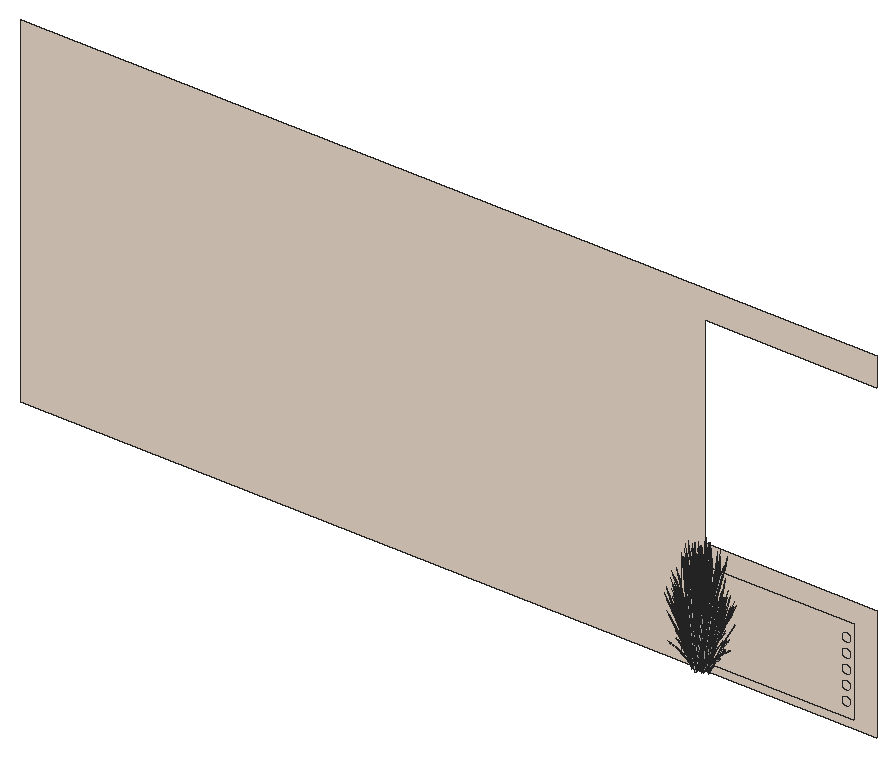
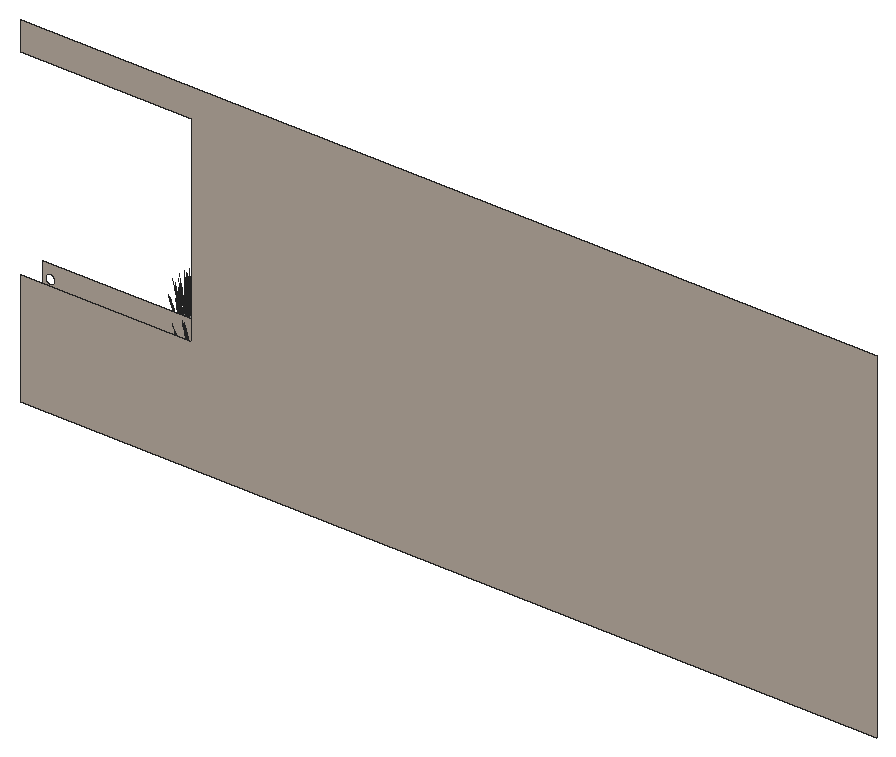
# SketchUp Ruby script. Lengths in inches.
U = 1.inch
M = Sketchup.active_model
def pt(a) = Geom::Point3d.new(a.map { |v| v * U })
def face(e, loops, mat)
  f = e.add_face(loops[0].map { |a| pt(a) })
  loops[1..].each { |l| e.add_face(l.map { |a| pt(a) }).erase! }
  f.material = f.back_material = mat if mat
  f
end
# faces: each face lists its corners as indices into pts; further lists are holes
def faces(e, pts, list, mat = nil) = list.each { |f| face(e, (f[0].is_a?(Array) ? f : [f]).map { |l| l.map { |i| pts[i] } }, mat) }
# xy, xz, yz: faces in a plane at the given z, y or x. An outline is a flat list of corners, or four numbers for a rectangle; further outlines are holes
def ring(l) = l.size == 4 ? [[l[0], l[1]], [l[2], l[1]], [l[2], l[3]], [l[0], l[3]]] : l.each_slice(2).to_a
def flat(e, list, mat, &to3) = list.each { |f| face(e, (f[0].is_a?(Array) ? f : [f]).map { |l| ring(l).map { |u, v| to3.(u, v) } }, mat) }
def xy(e, z, list, mat = nil) = flat(e, list, mat) { |x, y| [x, y, z] }
def xz(e, y, list, mat = nil) = flat(e, list, mat) { |x, z| [x, y, z] }
def yz(e, x, list, mat = nil) = flat(e, list, mat) { |y, z| [x, y, z] }
def lines(e, pts, list) = list.each { |a, b| e.add_line(pt(pts[a]), pt(pts[b])) }
# prism: a flat outline (further loops are holes) pulled along v
def prism(e, loops, v, mat = nil)
  f = face(e, loops, mat); d = Geom::Vector3d.new(v.map { |x| x * U })
  f.pushpull(f.normal.samedirection?(d) ? d.length : -d.length)
end
def box(e, o, s, mat = nil) = prism(e, [[o, [o[0] + s[0], o[1], o[2]], [o[0] + s[0], o[1] + s[1], o[2]], [o[0], o[1] + s[1], o[2]]]], [0, 0, s[2]], mat)
def at(x, y, z, deg = 0) = Geom::Transformation.translation(pt([x, y, z])) * Geom::Transformation.rotation(ORIGIN, Z_AXIS, deg.degrees)
def axes(o, x, y, z) = Geom::Transformation.new([*x, 0, *y, 0, *z, 0, *pt(o).to_a, 1])
def part(name) = M.definitions.add(name)
# library, detail: a bought-in or finely detailed component or shape, given as its bounding box
def library(name, o, s) = part(name).tap { |d| box(d.entities, o, s) }
def detail(e, o, s) = box(e.add_group.entities, o, s)
def put(e, d, t, mat = nil) = e.add_instance(d, t).tap { |i| i.material = mat if mat }
def group(e, t, mat = nil) = e.add_group.tap { |g| g.transformation = t; g.material = mat if mat }.entities
root = M.entities
M.materials.add("C01_Vanilla_Cream").color = [244, 228, 212]
M.materials.add("LightPink_Translucent").color = [144, 107, 117]
M.materials["LightPink_Translucent"].alpha = 0.75
c1 = part("blade")
p = [[2.15,0.21,22],[0,0.17,0],[0.09,0.45,0],[2.18,0.31,22],[2.29,0.31,22],[0.38,0.45,0],
  [2.48,0.24,33],[2.49,0.24,33],[2.48,0.22,33]]
faces(c1.entities,p,[[0,1,2,3],[4,5,2,3],[6,3,4,7],[8,0,3,6]])
c2 = part("seeds")
p = [[0.3,-0.1,1.38],[-0.01,-0.03,1.59],[-0.01,-0.03,0.03],[0.14,-0.07,-0.07],[0.29,-0.03,3],[0.15,0.01,3.11]]
faces(c2.entities,p,[[0,1,2,3],[1,0,4,5]],"LightPink_Translucent")
c3 = part("blade with seeds")
put(c3.entities,c1,at(0,0,0))
put(c3.entities,c2,axes([2.4,0.25,30.99],[1.5799,-0.05474,1.17369],[-0.12525,1.92788,0.29478],[-0.07173,-0.02425,1.56792]))
xz(root,468,[[[288,462,360,498],[357,490,356.48,490.07,356,490.27,355.59,490.59,355.27,491,355.07,491.48,355,492,355.07,492.52,355.27,493,355.59,493.41,356,493.73,356.48,493.93,357,494,357.52,493.93,358,493.73,358.41,493.41,358.73,493,358.93,492.52,359,492,358.93,491.48,358.73,491,358.41,490.59,358,490.27,357.52,490.07],[357,484,356.48,484.07,356,484.27,355.59,484.59,355.27,485,355.07,485.48,355,486,355.07,486.52,355.27,487,355.59,487.41,356,487.73,356.48,487.93,357,488,357.52,487.93,358,487.73,358.41,487.41,358.73,487,358.93,486.52,359,486,358.93,485.48,358.73,485,358.41,484.59,358,484.27,357.52,484.07],[357,478,356.48,478.07,356,478.27,355.59,478.59,355.27,479,355.07,479.48,355,480,355.07,480.52,355.27,481,355.59,481.41,356,481.73,356.48,481.93,357,482,357.52,481.93,358,481.73,358.41,481.41,358.73,481,358.93,480.52,359,480,358.93,479.48,358.73,479,358.41,478.59,358,478.27,357.52,478.07],[357,472,356.48,472.07,356,472.27,355.59,472.59,355.27,473,355.07,473.48,355,474,355.07,474.52,355.27,475,355.59,475.41,356,475.73,356.48,475.93,357,476,357.52,475.93,358,475.73,358.41,475.41,358.73,475,358.93,474.52,359,474,358.93,473.48,358.73,473,358.41,472.59,358,472.27,357.52,472.07],[357,466,356.48,466.07,356,466.27,355.59,466.59,355.27,467,355.07,467.48,355,468,355.07,468.52,355.27,469,355.59,469.41,356,469.73,356.48,469.93,357,470,357.52,469.93,358,469.73,358.41,469.41,358.73,469,358.93,468.52,359,468,358.93,467.48,358.73,467,358.41,466.59,358,466.27,357.52,466.07]]],"C01_Vanilla_Cream")
xz(root,480,[[0,450,0,594,360,594,360,582,288,582,288,498,360,498,360,450]],"C01_Vanilla_Cream")
put(root,c3,axes([303.38,460.31,465.51],[-0.14302,-0.44985,-0.38324],[0.54163,-0.07869,-0.29685],[0.15522,-0.12083,0.7333]))
put(root,c3,axes([301.01,458.76,463.6],[-0.38473,0.28263,-0.02919],[-0.35252,-0.30954,-0.13237],[-0.02482,-0.08771,0.43661]))
put(root,c3,axes([299.11,458.9,465.54],[-0.11979,-0.00348,1.31208],[-0.38137,0.34775,-0.2075],[-0.20349,-0.07106,0.10523]))
put(root,c3,axes([303.63,460.63,465.78],[-0.515,-0.27165,-0.0912],[0.2967,-0.3934,-0.50621],[0.1455,-0.13675,0.76918]))
put(root,c3,axes([301.51,462.11,464.49],[0.48111,0.19866,1.13446],[-0.47133,0.42798,0.44862],[-0.21112,-0.25366,0.95105]))
put(root,c3,axes([300.5,459.43,465.79],[0.08599,0.39682,0.2656],[-0.49155,0.10478,-0.3429],[-0.13203,-0.11372,0.65611]))
put(root,c3,axes([298.99,460.74,463.51],[0,-0.49266,-0.37238],[0.62289,0,0],[0,-0.11221,1.18128]))
put(root,c3,axes([300.72,459.28,463.51],[0.52105,-0.24633,-0.37238],[0.31144,0.44171,0],[0.11867,-0.0561,1.18128]))
put(root,c3,axes([303.8125,460.13,463.94],[-0.19889,-0.01459,1.07251],[-0.20376,-0.39145,-0.23066],[0.24434,-0.11074,0.45856]))
put(root,c3,axes([299.02,459.68,465.82],[0.45978,-0.36358,0.40322],[0.39653,0.38611,0.33247],[-0.21571,-0.06707,0.83437]))
put(root,c3,axes([304.9,460.51,465.53],[-0.07272,-0.00374,1.33037],[-0.30197,-0.40092,-0.12571],[0.12127,-0.13182,0.23543]))
put(root,c3,axes([301.34,460.29,463.54],[0.375,-0.3703,-0.46765],[0.46584,0.33578,-0.12274],[0.15027,-0.09237,1.03225]))
put(root,c3,axes([304.04,459.41,464.07],[-0.18544,0.25079,0.86145],[-0.15939,-0.33694,0.63294],[0.15316,-0.08443,0.18974]))
put(root,c3,axes([303.78,460.35,465.39],[0.48462,-0.07041,-0.2656],[0.12797,0.4025,0.3429],[0.13888,-0.10811,0.65611]))
put(root,c3,axes([299.23,459.68,465.55],[0.02803,-0.37463,0.04823],[0.42332,0.01027,0.37966],[-0.16216,-0.0392,0.57892]))
put(root,c3,axes([300.6875,460.9375,463.66],[0.27012,-0.44393,-0.33554],[0.56127,0.21365,0.16149],[0,-0.10233,1.07733]))
put(root,c3,axes([299.07,459.8,465.39],[-0.31678,-0.30846,-0.2656],[0.36171,-0.29199,0.3429],[-0.18378,-0.04443,0.65611]))
put(root,c3,axes([300.93,460.72,464],[-0.06488,-0.56215,-0.21822],[0.6757,-0.03399,-0.37502],[0.11898,-0.07488,1.19781]))
put(root,c3,axes([299.26,460.75,463.52],[0.38863,-0.30738,-0.23233],[0.38863,0.30738,0.23233],[0,-0.09901,1.0423]))
put(root,c3,axes([299.1,459.27,463.6],[-0.1606,0.40228,-0.02919],[-0.4943,-0.12375,-0.13237],[-0.07505,-0.0658,0.43661]))
put(root,c3,axes([303.38,460.59,465.79],[-0.48462,0.07041,0.2656],[-0.12797,-0.4025,-0.3429],[0.13888,-0.10811,0.65611]))
put(root,c3,axes([300.62,461.31,464],[-0.62699,-0.23507,-0.21822],[0.3019,-0.49615,-0.37502],[-0.0197,-0.12182,1.19781]))
put(root,c3,axes([298.83,461.11,463.78],[-0.69617,0,0],[0,-0.55062,-0.38706],[0,-0.12541,1.22783]))
put(root,c3,axes([298.95,460.13,463.94],[0.1087,0.13716,1.07251],[-0.25048,0.37284,-0.23066],[-0.25719,-0.08912,0.45856]))
put(root,c3,axes([300.84,459.47,463.52],[0.51941,0.1219,-0.23233],[-0.13078,0.42928,0.23233],[0.10471,-0.0495,1.0423]))
put(root,c3,axes([299.4,460.01,465.74],[-0.55654,-0.01186,-0.53284],[0.03738,-0.49951,0.0643],[-0.23578,-0.05271,0.75375]))
put(root,c3,axes([303.82,460.53,465.55],[0.3822,0.20719,0.04823],[-0.22252,0.29505,0.37966],[0.12254,-0.09539,0.57892]))
put(root,c3,axes([303.71,460.44,465.55],[0.13808,0.45342,0.36002],[-0.54163,0.07869,0.29685],[0.15963,-0.10664,0.74497]))
put(root,c3,axes([305.18,460.99,465.54],[0.07726,-0.07504,1.31208],[-0.09888,-0.46032,-0.2075],[0.19384,-0.08728,0.10523]))
put(root,c3,axes([299.375,460.97,463.75],[-0.51786,0.4142,0.23067],[-0.51817,-0.40984,-0.27369],[-0.01808,-0.11762,1.23664]))
put(root,c3,axes([298.65,459.19,465.53],[0.04127,0.04917,1.33037],[-0.19898,0.44196,-0.12571],[-0.20151,0.0032,0.23543]))
put(root,c3,axes([301.02,461.16,463.82],[0.6273,0.23878,0.18048],[-0.3019,0.49615,0.37502],[0,-0.11437,1.20407]))
put(root,c3,axes([300.78,461.83,463.83],[0.14756,-0.58378,-0.17572],[0.69966,0.10176,0.38453],[-0.12225,-0.08062,1.1733]))
put(root,c3,axes([299.22,460.11,465.51],[-0.40426,0.32635,-0.38324],[-0.35404,-0.34474,-0.29685],[-0.2054,-0.04965,0.7333]))
put(root,c3,axes([299.52,459.96,465.79],[0.31678,0.30846,0.2656],[-0.36171,0.29199,-0.3429],[-0.18378,-0.04443,0.65611]))
put(root,c3,axes([298.31,460.54,464.07],[0.35544,-0.03525,0.86145],[-0.22547,0.31061,0.63294],[-0.17565,-0.04659,0.18974]))
put(root,c3,axes([300.82,460.83,464.04],[-0.60457,0.03041,0.33554],[-0.05467,-0.50484,-0.16149],[0.10823,-0.05117,1.07733]))
put(root,c3,axes([299.43,459.76,465.78],[-0.02981,0.50103,-0.0912],[-0.56442,-0.01369,-0.50621],[-0.21738,-0.0348,0.76918]))
put(root,c3,axes([299.26,461.19,463.86],[0,0.49266,0.37238],[-0.62289,0,0],[0,-0.11221,1.18128]))
put(root,c3,axes([303.65,461.6875,465.78],[-0.28012,-0.44611,-0.0912],[0.49717,-0.21923,-0.50621],[0.20951,-0.05886,0.76918]))
put(root,c3,axes([303.63,461.3,465.51],[0.15083,-0.44814,-0.38324],[0.51712,0.15361,-0.29685],[0.2082,-0.04109,0.7333]))
put(root,c3,axes([302.8125,459.48,463.78],[0.34808,-0.49367,0],[0.58235,0.27531,-0.38706],[0.13264,0.0627,1.22783]))
put(root,c3,axes([298.71,460.45,464.91],[0.23093,-0.01116,1.28532],[-0.15319,0.4836,0.10393],[-0.32909,-0.02991,0.54946]))
put(root,c3,axes([300.73,461.59,463.66],[-0.33445,-0.41351,-0.33554],[0.50659,-0.29119,0.16149],[-0.10823,-0.05117,1.07733]))
put(root,c3,axes([300.8,461.01,463.77],[0.24206,0.5509,0.34316],[-0.69162,0.19157,0.13466],[0.00845,-0.10123,1.19142]))
put(root,c3,axes([304.18,461.43,463.49],[-0.35858,0.05912,1.06187],[-0.05708,-0.47061,0.06078],[0.25115,-0.07123,0.60425]))
put(root,c3,axes([304.83,461.01,463.7],[-0.34516,-0.31503,-0.04866],[0.37803,-0.28865,-0.22062],[0.10711,-0.02032,0.72768]))
put(root,c3,axes([300.68,461.44,464.04],[-0.27012,0.44393,0.33554],[-0.56127,-0.21365,-0.16149],[0,-0.10233,1.07733]))
put(root,c3,axes([301.67,461.05,463.65],[0,-0.57005,0],[0.69617,0,0],[0,0,1.34592]))
put(root,c3,axes([302.51,459.74,463.86],[-0.52105,-0.24633,0.37238],[0.31144,-0.44171,0],[0.11867,0.0561,1.18128]))
put(root,c3,axes([303.53,461.47,465.74],[0.48922,-0.21758,-0.53284],[0.27264,0.44789,0.0643],[0.23638,-0.05088,0.75375]))
put(root,c3,axes([300.43,461.75,463.54],[-0.57914,-0.08077,-0.46765],[0.12221,-0.49823,-0.12274],[-0.17283,-0.06037,1.03225]))
put(root,c3,axes([301.34,460.7,463.77],[-0.46162,0.4471,0.34316],[-0.54842,-0.39467,0.13466],[0.11129,-0.04462,1.19142]))
put(root,c3,axes([301.84,461.5,463.72],[-0.51786,-0.42404,-0.04598],[0.51817,-0.4243,0],[-0.01808,-0.01481,1.31678]))
put(root,c3,axes([300.54,459.96,463.86],[-0.16083,0.48962,0.13232],[-0.58854,-0.13856,0.26315],[0.10167,-0.00238,1.20305]))
put(root,c3,axes([303.46,461.55,465.79],[-0.46269,-0.13744,0.2656],[0.13495,-0.40096,-0.3429],[0.18628,-0.03677,0.65611]))
put(root,c3,axes([298.62,460.82,465.55],[0.15729,-0.44921,0.36002],[0.51712,0.15361,0.29685],[-0.20336,0.027,0.74497]))
put(root,c3,axes([300.29,460.35,463.2],[-0.548,0.19724,0.96696],[-0.17442,-0.56594,0.37572],[0.3365,0.00941,1.09981]))
put(root,c3,axes([301.77,460.5,463.96],[0.1074,-0.43968,0.1086],[0.52474,0.07632,-0.3101],[0.0955,0.04515,0.95058]))
put(root,c3,axes([298.58,460.7,465.55],[-0.20448,-0.33592,0.04823],[0.37288,-0.16442,0.37966],[-0.16437,0.03244,0.57892]))
put(root,c3,axes([300.86,461.55,463.77],[0.70367,0.1038,0.34316],[-0.1432,0.58624,0.13466],[-0.10283,-0.05661,1.19142]))
put(root,c3,axes([304.57,461.125,463.12],[-0.0291,-0.0748,1.32257],[0.20181,-0.43752,-0.20205],[0.20357,-0.00629,0.22528]))
put(root,c3,axes([298.57,461.05,463.12],[0.01412,0.07764,1.32257],[-0.28464,0.40547,-0.20205],[-0.20218,-0.02044,0.22528]))
put(root,c3,axes([301.54,460.62,464.04],[-0.33445,-0.41351,0.33554],[0.50659,-0.29119,-0.16149],[0.10823,0.05117,1.07733]))
put(root,c3,axes([299.8125,462.51,463.52],[-0.13078,-0.42928,-0.23233],[0.51941,-0.1219,0.23233],[-0.10471,-0.0495,1.0423]))
put(root,c3,axes([300.48,462.48,463.86],[0.59825,-0.13076,0.13232],[0.14773,0.48663,0.26315],[-0.05336,-0.0709,1.20305]))
put(root,c3,axes([301.71,460.65,464],[0.56211,-0.32708,-0.21822],[0.3738,0.46216,-0.37502],[0.13869,0.04694,1.19781]))
put(root,c3,axes([303.95,461.51,465.39],[0.46269,0.13744,-0.2656],[-0.13495,0.40096,0.3429],[0.18628,-0.03677,0.65611]))
put(root,c3,axes([299.67,462.69,463.51],[-0.52105,-0.24633,-0.37238],[0.31144,-0.44171,0],[-0.11867,-0.0561,1.18128]))
put(root,c3,axes([303.13,459.78,463.51],[0.52105,0.24633,-0.37238],[-0.31144,0.44171,0],[0.11867,0.0561,1.18128]))
put(root,c3,axes([298.51,460.87,465.39],[-0.46269,-0.13744,-0.2656],[0.13495,-0.40096,0.3429],[-0.18628,0.03677,0.65611]))
put(root,c3,axes([302.14,461.18,463.65],[0.62289,0,0],[0,0.51004,0],[0,0,1.33805]))
put(root,c3,axes([301.08,461.82,464],[-0.56211,0.32708,-0.21822],[-0.3738,-0.46216,-0.37502],[-0.13869,-0.04694,1.19781]))
put(root,c3,axes([302.32,459.99,463.86],[-0.59825,0.13076,0.13232],[-0.14773,-0.48663,0.26315],[0.05336,0.0709,1.20305]))
put(root,c3,axes([302.6875,461.01,464.91],[-0.23093,0.01116,1.28532],[0.15319,-0.4836,0.10393],[0.32909,0.02991,0.54946]))
put(root,c3,axes([302.98,459.96,463.52],[0.13078,0.42928,-0.23233],[-0.51941,0.1219,0.23233],[0.10471,0.0495,1.0423]))
put(root,c3,axes([303.88,461.68,465.55],[0.20448,0.33592,0.04823],[-0.37288,0.16442,0.37966],[0.16437,-0.03244,0.57892]))
put(root,c3,axes([301.9375,460.92,463.79],[-0.70367,-0.1038,0.36899],[0.1432,-0.58624,0.1448],[0.10283,0.05661,1.2811]))
put(root,c3,axes([303.84,461.56,465.55],[-0.15729,0.44921,0.36002],[-0.51712,-0.15361,0.29685],[0.20336,-0.027,0.74497]))
put(root,c3,axes([301.38,462.37,463.65],[-0.18165,-0.42474,0],[0.51872,-0.14874,0],[0,0,1.15778]))
put(root,c3,axes([301.03,461.97,463.96],[-0.1074,0.43968,0.1086],[-0.52474,-0.07632,-0.3101],[-0.0955,-0.04515,0.95058]))
put(root,c3,axes([299,460.83,465.79],[0.46269,0.13744,0.2656],[-0.13495,0.40096,-0.3429],[-0.18628,0.03677,0.65611]))
put(root,c3,axes([302.06,462.31,463.64],[0.5845,-0.16716,-0.14398],[0.20539,0.48152,0.00006],[0.06452,-0.01848,1.30423]))
put(root,c3,axes([302.26,462.51,463.86],[0.16083,-0.48962,0.13232],[0.58854,0.13856,0.26315],[-0.10167,0.00238,1.20305]))
put(root,c3,axes([302.125,461.4,463.66],[0.38863,0.31822,0],[-0.38863,0.31822,0],[0,0,1.2695]))
put(root,c3,axes([299.92,460.8,464.51],[0.15825,-0.07127,1.32798],[0.05457,0.4976,0.10393],[-0.34278,0.06603,0.47463]))
put(root,c3,axes([303.18,461.26,463.86],[-0.43742,-0.35886,0.13232],[0.44081,-0.34807,0.26315],[-0.04831,0.07329,1.20305]))
put(root,c3,axes([302.37,460.72,463.54],[0.57914,0.08077,-0.46765],[-0.12221,0.49823,-0.12274],[0.17283,0.06037,1.03225]))
put(root,c3,axes([304.93,461.59,464.07],[-0.34399,0.08133,0.86145],[0.16192,-0.33614,0.63294],[0.18249,0.023,0.18974]))
put(root,c3,axes([301.25,462.5625,463.65],[-0.56127,-0.22118,0],[0.27012,-0.45959,0],[0,0,1.2203]))
put(root,c3,axes([301.72,461.97,463.85],[-0.54364,-0.39653,-0.18894],[0.45745,-0.44527,0.41347],[-0.14639,0.04639,1.26162]))
put(root,c3,axes([300.28,462.73,463.86],[0.52105,0.24633,0.37238],[-0.31144,0.44171,0],[-0.11867,-0.0561,1.18128]))
put(root,c3,axes([302.12,461.03,464.04],[0.27012,-0.44393,0.33554],[0.56127,0.21365,-0.16149],[0,0.10233,1.07733]))
put(root,c3,axes([304.77,463.01,465.53],[-0.05034,-0.04313,1.33037],[0.11012,-0.46232,-0.12571],[0.1983,-0.02954,0.23543]))
put(root,c3,axes([298.22,461.14,465.54],[-0.09091,0.06396,1.31208],[0.00773,0.46734,-0.2075],[-0.20839,0.06078,0.10523]))
put(root,c3,axes([302.02,461.28,463.72],[0,0.56976,-0.04228],[-0.69617,0,0],[0,0.01791,1.34526]))
put(root,c3,axes([298.83,461.07,465.51],[-0.15083,0.44814,-0.38324],[-0.51712,-0.15361,-0.29685],[-0.2082,0.04109,0.7333]))
put(root,c3,axes([298.8,460.69,465.78],[0.28012,0.44611,-0.0912],[-0.49717,0.21923,-0.50621],[-0.20951,0.05886,0.76918]))
put(root,c3,axes([302.07,460.88,463.66],[0.33445,0.41351,-0.33554],[-0.50659,0.29119,0.16149],[0.10823,0.05117,1.07733]))
put(root,c3,axes([304.33,462.625,464.95],[-0.10656,-0.41414,-0.02619],[0.50364,-0.09521,-0.11874],[0.10517,0.02626,0.39164]))
put(root,c3,axes([299.98,462.99,463.78],[-0.34808,0.49367,0],[-0.58235,-0.27531,-0.38706],[-0.13264,-0.0627,1.22783]))
put(root,c3,axes([303.02,462.61,465.78],[0.02981,-0.50103,-0.0912],[0.56442,0.01369,-0.50621],[0.21738,0.0348,0.76918]))
put(root,c3,axes([303.54,461.28,463.86],[0,-0.49266,0.37238],[0.62289,0,0],[0,0.11221,1.18128]))
put(root,c3,axes([301.98,461.64,464.04],[0.60457,-0.03041,0.33554],[0.05467,0.50484,-0.16149],[-0.10823,0.05117,1.07733]))
put(root,c3,axes([302.36,461.13,463.96],[0.51872,-0.14368,0.1086],[0.18165,0.41027,-0.3101],[0,0.09029,0.95058]))
put(root,c3,axes([302.9375,462.42,465.79],[-0.31678,-0.30846,0.2656],[0.36171,-0.29199,-0.3429],[0.18378,0.04443,0.65611]))
put(root,c3,axes([301.44,461.89,463.66],[-0.60457,0.03041,-0.33554],[-0.05467,-0.50484,0.16149],[-0.10823,0.05117,1.07733]))
put(root,c3,axes([304.28,462.13,463.94],[-0.13408,-0.12117,1.07251],[0.17446,-0.40083,-0.23066],[0.27128,0.0543,0.45856]))
put(root,c3,axes([301.89,462.57,463.65],[0.56127,0.22118,0],[-0.27012,0.45959,0],[0,0,1.31215]))
put(root,c3,axes([303.52,462.3125,465.54],[0.11943,-0.00833,1.31208],[0.32759,-0.38275,-0.2075],[0.21244,0.05052,0.10523]))
put(root,c3,axes([302.11,463.06,463.64],[-0.34375,-0.4954,-0.03857],[0.58235,-0.27531,0.38706],[-0.1435,0.04717,1.22723]))
put(root,c3,axes([301.99,461.86,463.96],[0.41131,0.296,0.1086],[-0.34309,0.33395,-0.3101],[-0.0955,0.04515,0.95058]))
put(root,c3,axes([298.74,461.9375,465.55],[-0.13808,-0.45342,0.36002],[0.54163,-0.07869,0.29685],[-0.15963,0.10664,0.74497]))
put(root,c3,axes([298.63,461.85,465.55],[-0.3822,-0.20719,0.04823],[0.22252,-0.29505,0.37966],[-0.12254,0.09539,0.57892]))
put(root,c3,axes([298.81,461.31,464.91],[0.19317,-0.10421,1.28532],[0.16263,0.48153,0.10393],[-0.30326,0.10883,0.54946]))
put(root,c3,axes([303.05,462.375,465.74],[0.55654,0.01186,-0.53284],[-0.03738,0.49951,0.0643],[0.23578,0.05271,0.75375]))
put(root,c3,axes([302.43,462.77,463.86],[0.52105,-0.24633,0.37238],[0.31144,0.44171,0],[-0.11867,0.0561,1.18128]))
put(root,c3,axes([301.68,462.38,463.72],[0.24206,0.56598,-0.04509],[-0.69162,0.19832,0],[0.00845,0.01976,1.2913]))
put(root,c3,axes([301.95,463,463.52],[-0.51941,-0.1219,-0.23233],[0.13078,-0.42928,0.23233],[-0.10471,0.0495,1.0423]))
put(root,c3,axes([298.21,462.125,463.94],[0.19348,0.04044,1.07251],[0.1247,0.41309,-0.23066],[-0.26282,0.07733,0.45856]))
put(root,c3,axes([299.07,461.79,465.79],[0.48462,-0.07041,0.2656],[0.12797,0.4025,-0.3429],[-0.13888,0.10811,0.65611]))
put(root,c3,axes([303.96,461.36,463.78],[0.69617,0,0],[0,0.55062,-0.38706],[0,0.12541,1.22783]))
put(root,c3,axes([297.21,461.61,465.53],[0.07105,0.01321,1.33037],[0.2198,0.43529,-0.12571],[-0.14545,0.11425,0.23543]))
put(root,c3,axes([303.68,461.64,463.65],[-0.69582,-0.00394,-0.03732],[0,-0.55062,0.37457],[-0.02187,0.12535,1.18764]))
put(root,c3,axes([302.18,461.16,464],[0.62699,0.23507,-0.21822],[-0.3019,0.49615,-0.37502],[0.0197,0.12182,1.19781]))
put(root,c3,axes([297.8,462.99,464.07],[0.23202,-0.22328,0.86145],[0.09155,0.35348,0.63294],[-0.16768,0.06329,0.18974]))
put(root,c3,axes([303.39,462.58,465.39],[0.31678,0.30846,-0.2656],[-0.36171,0.29199,0.3429],[0.18378,0.04443,0.65611]))
put(root,c3,axes([303.54,461.72,463.52],[-0.38863,0.30738,-0.23233],[-0.38863,-0.30738,0.23233],[0,0.09901,1.0423]))
put(root,c3,axes([301.86,461.75,464],[0.06488,0.56215,-0.21822],[-0.6757,0.03399,-0.37502],[-0.11898,0.07488,1.19781]))
put(root,c3,axes([303.23,462.7,465.55],[-0.02803,0.37463,0.04823],[-0.42332,-0.01027,0.37966],[0.16216,0.0392,0.57892]))
put(root,c3,axes([302.11,461.53,463.66],[-0.27012,0.44393,-0.33554],[-0.56127,-0.21365,0.16149],[0,0.10233,1.07733]))
put(root,c3,axes([298.68,462.03,465.39],[-0.48462,0.07041,-0.2656],[-0.12797,-0.4025,0.3429],[-0.13888,0.10811,0.65611]))
put(root,c3,axes([303.26,462.58,465.55],[-0.41051,0.32462,0.36002],[-0.35404,-0.34474,0.29685],[0.1926,0.05988,0.74497]))
put(root,c3,axes([297.97,462.93,466.23],[0.49129,0.13151,-0.04866],[-0.15113,0.40475,-0.22062],[-0.08035,0.06145,0.72768]))
put(root,c3,axes([301.46,462.18,463.54],[-0.375,0.3703,-0.46765],[-0.46584,-0.33578,-0.12274],[-0.15027,0.09237,1.03225]))
put(root,c3,axes([301.96,462.95,465.79],[-0.08599,-0.39682,0.2656],[0.49155,-0.10478,-0.3429],[0.13203,0.11372,0.65611]))
put(root,c3,axes([302.125,462.81,463.75],[0.697,0.16013,0.23067],[-0.17437,0.57237,-0.27369],[-0.11536,0.07164,1.23664]))
put(root,c3,axes([302.08,463.19,463.51],[-0.52105,0.24633,-0.37238],[-0.31144,-0.44171,0],[-0.11867,0.0561,1.18128]))
put(root,c3,axes([303.81,461.73,463.51],[0,0.49266,-0.37238],[-0.62289,0,0],[0,0.11221,1.18128]))
put(root,c3,axes([302.25,461.79,464.91],[-0.2068,-0.08488,1.28532],[0.42797,-0.35609,0.10393],[0.26673,0.16064,0.54946]))
put(root,c3,axes([302.29,460.67,465.36],[-0.48108,-0.25598,1.03712],[0.50798,-0.39855,0.44749],[0.15521,0.24018,1.00248]))
put(root,c3,axes([298.82,461.75,465.78],[0.515,0.27165,-0.0912],[-0.2967,0.3934,-0.50621],[-0.1455,0.13675,0.76918]))
put(root,c3,axes([303.02,462.76,464.07],[-0.31347,-0.14166,0.86145],[0.40476,-0.14393,0.63294],[0.10917,0.12192,0.18974]))
put(root,c3,axes([301.91,463.16,465.78],[0.33176,-0.4217,-0.0912],[0.48044,0.24295,-0.50621],[0.16701,0.11914,0.76918]))
put(root,c3,axes([299.51,461.63,464.91],[0.13906,-0.15138,1.28532],[0.35111,0.40859,0.10393],[-0.24082,0.18608,0.54946]))
put(root,c3,axes([299.08,462.07,465.51],[0.14302,0.44985,-0.38324],[-0.54163,0.07869,-0.29685],[-0.15522,0.12083,0.7333]))
put(root,c3,axes([299.73,462.59,465.79],[0.3767,-0.25939,0.2656],[0.3566,0.29618,-0.3429],[-0.05426,0.15048,0.65611]))
put(root,c3,axes([302.55,463.12,463.78],[0.34808,0.49367,0],[-0.58235,0.27531,-0.38706],[-0.13264,0.0627,1.22783]))
put(root,c3,axes([301.48,463.51,465.53],[0.00165,-0.05965,1.33037],[0.47711,-0.26315,-0.12571],[0.16572,0.09393,0.23543]))
put(root,c3,axes([303.1,463.28,463.12],[0.04056,-0.07113,1.32257],[0.51066,-0.20948,-0.20205],[0.15482,0.10842,0.22528]))
put(root,c3,axes([302.25,461.16,464.13],[-0.01521,-0.46386,1.05954],[0.68831,0.12024,0.44862],[-0.1628,0.25382,1.00012]))
put(root,c3,axes([302.43,461.67,463.57],[0.20414,0.45107,-0.51909],[-0.58805,0.16245,-0.13624],[0.02256,0.15274,1.1458]))
put(root,c3,axes([299.39,462.83,465.55],[-0.45752,-0.02296,0.04823],[0.01254,-0.34663,0.37966],[-0.04787,0.13278,0.57892]))
put(root,c3,axes([298.41,463.22,463.12],[0.07468,0.04922,1.32257],[0.12663,0.45605,-0.20205],[-0.16551,0.09725,0.22528]))
put(root,c3,axes([299.53,462.86,465.55],[-0.39645,-0.33614,0.36002],[0.42102,-0.2899,0.29685],[-0.07313,0.15771,0.74497]))
put(root,c3,axes([302.31,462.95,465.51],[0.54938,-0.11711,-0.38324],[0.0961,0.44351,-0.29685],[0.14756,0.1271,0.7333]))
put(root,c3,axes([300.78,463.02,465.79],[0.16784,-0.37886,0.2656],[0.48968,0.1105,-0.3429],[0.0449,0.15254,0.65611]))
put(root,c3,axes([303.06,463.4,464],[-0.35702,-0.01545,0.78795],[0.23577,-0.32816,0.43504],[0.14104,0.11659,0.61808]))
put(root,c3,axes([302.04,463.3125,465.55],[-0.25304,0.31296,0.04823],[-0.36033,-0.18221,0.37966],[0.11649,0.10034,0.57892]))
put(root,c3,axes([301.44,464.37,466.23],[0.38473,-0.28263,-0.04866],[0.35252,0.30954,-0.22062],[0.02482,0.08771,0.72768]))
put(root,c3,axes([302.14,463.23,465.55],[-0.55374,0.11306,0.36002],[-0.0961,-0.44351,0.29685],[0.13023,0.13071,0.74497]))
put(root,c3,axes([299.41,462,464.91],[0.10366,-0.16934,1.28532],[0.43488,0.35044,0.10393],[-0.19618,0.21841,0.54946]))
put(root,c3,axes([301.9,462.6,463.94],[0.00982,-0.16331,1.07251],[0.4695,-0.18242,-0.23066],[0.14493,0.19547,0.45856]))
put(root,c3,axes([300.63,463.36,465.55],[-0.41024,0.16744,0.04823],[-0.2008,-0.30532,0.37966],[0.03962,0.13459,0.57892]))
put(root,c3,axes([299.53,462.96,465.39],[-0.3767,0.25939,-0.2656],[-0.3566,-0.29618,0.3429],[-0.05426,0.15048,0.65611]))
put(root,c3,axes([298.23,462.88,465.54],[-0.01384,0.09749,1.31208],[0.39274,0.33916,-0.2075],[-0.10282,0.16039,0.10523]))
put(root,c3,axes([299.49,462.66,466.05],[0.61188,0.02441,-0.10123],[-0.01672,0.46217,-0.56189],[-0.0425,0.178,0.85379]))
put(root,c3,axes([300.62,463.18,465.78],[0.54481,-0.22937,-0.0912],[0.26773,0.4071,-0.50621],[0.07188,0.17155,0.76918]))
put(root,c3,axes([300.78,463.33,465.8],[-0.54859,-0.1288,0.39962],[0.18759,-0.42344,0.32951],[0.03297,0.16652,0.82692]))
put(root,c3,axes([299.77,463.97,464.07],[-0.01441,-0.29294,0.86145],[0.36003,0.20894,0.63294],[-0.07081,0.13963,0.18974]))
put(root,c3,axes([300.72,463.27,463.12],[0.0901,-0.02681,1.32257],[0.54199,0.14755,-0.20205],[0.01585,0.1663,0.22528]))
put(root,c3,axes([299.9,462.84,465.75],[0.39855,0.33102,-0.4254],[-0.42102,0.2899,-0.32951],[-0.06064,0.16819,0.81396]))
put(root,c3,axes([299.47,463.33,464.12],[0.50577,-0.08724,0.04881],[0.11627,0.35148,-0.64728],[-0.03206,0.17792,0.5802]))
put(root,c3,axes([301.09,463.16,465.51],[0.54728,0.1235,-0.38324],[-0.18759,0.42344,-0.29685],[0.05018,0.17048,0.7333]))
put(root,c3,axes([301.4,462.28,464.91],[-0.12726,-0.15818,1.28532],[0.58807,-0.13317,0.10393],[0.13291,0.24832,0.54946]))
put(root,c3,axes([300.84,463.42,465.39],[-0.16784,0.37886,-0.2656],[-0.48968,-0.1105,0.3429],[0.0449,0.15254,0.65611]))
put(root,c3,axes([299.78,462.68,466],[-0.01449,0.45571,-0.59145],[-0.61002,-0.03061,0.07138],[-0.06438,0.19306,0.83667]))
put(root,c3,axes([298.1875,463.88,465.53],[0.06316,-0.02974,1.33037],[0.52204,0.19785,-0.12571],[-0.01227,0.16473,0.23543]))
put(root,c3,axes([300.36,462.36,464.91],[-0.01363,-0.18909,1.28532],[0.5906,0.12544,0.10393],[-0.03653,0.26947,0.54946]))
put(root,c3,axes([300.89,463.08,465.74],[0.26572,0.40059,-0.53284],[-0.54698,0.22325,0.0643],[0.06214,0.19355,0.75375]))
put(root,c3,axes([299.35,463.71,463.94],[0.17569,-0.07772,1.07251],[0.43377,0.23434,-0.23066],[-0.12911,0.20277,0.45856]))
put(root,c3,axes([300.49,464.09,465.54],[0.07057,0.07933,1.31208],[0.56952,0.03117,-0.2075],[0.05727,0.17496,0.10523]))
put(root,c3,axes([299.58,463.33,464.52],[0.01223,-0.25433,1.15759],[0.55017,0.13434,0.15997],[-0.04767,0.27105,0.54661]))
